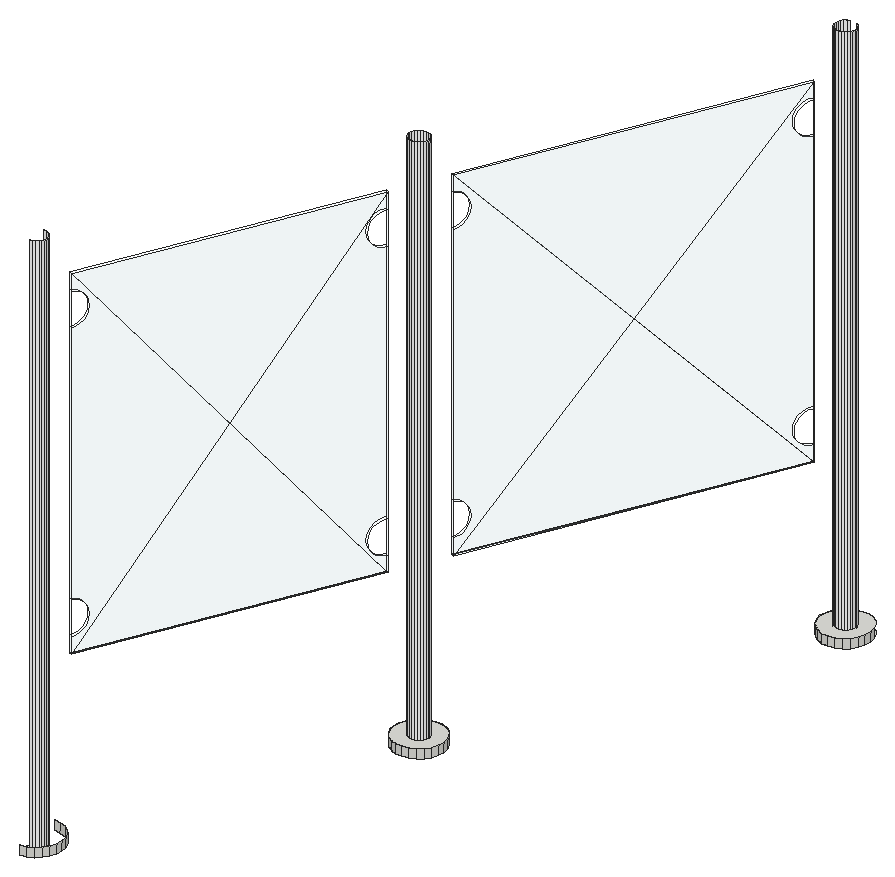
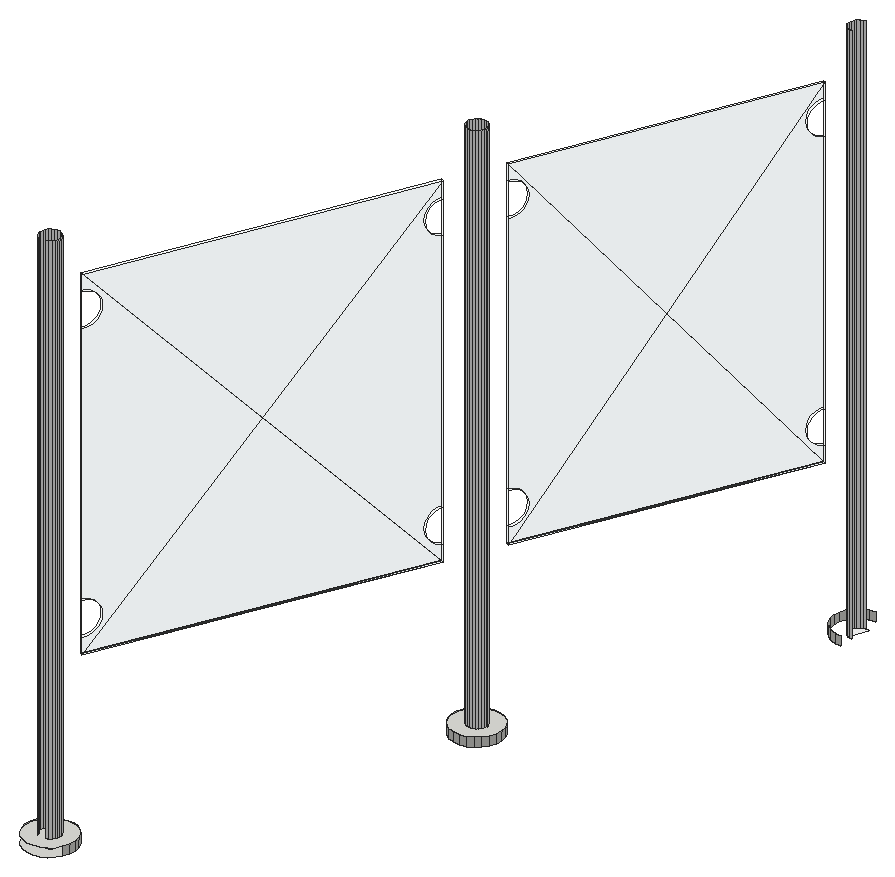
# SketchUp Ruby script. Lengths in inches.
U = 1.inch
M = Sketchup.active_model
def pt(a) = Geom::Point3d.new(a.map { |v| v * U })
def face(e, loops, mat)
  f = e.add_face(loops[0].map { |a| pt(a) })
  loops[1..].each { |l| e.add_face(l.map { |a| pt(a) }).erase! }
  f.material = f.back_material = mat if mat
  f
end
# faces: each face lists its corners as indices into pts; further lists are holes
def faces(e, pts, list, mat = nil) = list.each { |f| face(e, (f[0].is_a?(Array) ? f : [f]).map { |l| l.map { |i| pts[i] } }, mat) }
# xy, xz, yz: faces in a plane at the given z, y or x. An outline is a flat list of corners, or four numbers for a rectangle; further outlines are holes
def ring(l) = l.size == 4 ? [[l[0], l[1]], [l[2], l[1]], [l[2], l[3]], [l[0], l[3]]] : l.each_slice(2).to_a
def flat(e, list, mat, &to3) = list.each { |f| face(e, (f[0].is_a?(Array) ? f : [f]).map { |l| ring(l).map { |u, v| to3.(u, v) } }, mat) }
def xy(e, z, list, mat = nil) = flat(e, list, mat) { |x, y| [x, y, z] }
def xz(e, y, list, mat = nil) = flat(e, list, mat) { |x, z| [x, y, z] }
def yz(e, x, list, mat = nil) = flat(e, list, mat) { |y, z| [x, y, z] }
def lines(e, pts, list) = list.each { |a, b| e.add_line(pt(pts[a]), pt(pts[b])) }
# prism: a flat outline (further loops are holes) pulled along v
def prism(e, loops, v, mat = nil)
  f = face(e, loops, mat); d = Geom::Vector3d.new(v.map { |x| x * U })
  f.pushpull(f.normal.samedirection?(d) ? d.length : -d.length)
end
def box(e, o, s, mat = nil) = prism(e, [[o, [o[0] + s[0], o[1], o[2]], [o[0] + s[0], o[1] + s[1], o[2]], [o[0], o[1] + s[1], o[2]]]], [0, 0, s[2]], mat)
def at(x, y, z, deg = 0) = Geom::Transformation.translation(pt([x, y, z])) * Geom::Transformation.rotation(ORIGIN, Z_AXIS, deg.degrees)
def axes(o, x, y, z) = Geom::Transformation.new([*x, 0, *y, 0, *z, 0, *pt(o).to_a, 1])
def part(name) = M.definitions.add(name)
# library, detail: a bought-in or finely detailed component or shape, given as its bounding box
def library(name, o, s) = part(name).tap { |d| box(d.entities, o, s) }
def detail(e, o, s) = box(e.add_group.entities, o, s)
def put(e, d, t, mat = nil) = e.add_instance(d, t).tap { |i| i.material = mat if mat }
def group(e, t, mat = nil) = e.add_group.tap { |g| g.transformation = t; g.material = mat if mat }.entities
root = M.entities
M.materials.add("Glass_Safety_01").color = [204, 235, 244]
M.materials["Glass_Safety_01"].alpha = 0.1
M.materials.add("[Color_000]").color = [255, 255, 255]
xy(root,321.27,[[[898.23,660.375,898.63,660.46,899,660.64,899.31,660.92,899.53,661.26,899.66,661.65,899.6875,662.06,899.61,662.46,899.42,662.83,899.15,663.14,898.81,663.36,898.74,663.38,898.42,663.49,898,663.52,897.6,663.43,897.23,663.25,896.93,662.98,896.7,662.63,896.57,662.24,896.55,661.83,896.63,661.43,896.8125,661.0625,897.09,660.76,897.43,660.53,897.82,660.4],[898.16,661.32,898,661.33,897.87,661.37,897.84,661.38,897.7,661.47,897.6,661.59,897.52,661.74,897.49,661.9,897.5,662.07,897.55,662.22,897.64,662.36,897.76,662.47,897.91,662.54,898.07,662.58,898.24,662.57,898.37,662.52,898.39,662.51,898.53,662.42,898.64,662.3,898.71,662.15,898.75,661.99,898.74,661.83,898.68,661.67,898.59,661.53,898.47,661.43,898.32,661.35]],[897.49,660.51,897.87,661.37,897.84,661.38,897.7,661.47,897.6,661.59,897.52,661.74,897.49,661.9,897.5,662.07,897.55,662.22,897.64,662.36,897.76,662.47,897.91,662.54,898.07,662.58,898.24,662.57,898.37,662.52,898.74,663.38,898.42,663.49,898,663.52,897.6,663.43,897.23,663.25,896.93,662.98,896.7,662.63,896.57,662.24,896.55,661.83,896.63,661.43,896.8125,661.0625,897.09,660.76,897.43,660.53],[897.87,661.37,898.37,662.52,898.24,662.57,898.07,662.58,897.91,662.54,897.76,662.47,897.64,662.36,897.55,662.22,897.5,662.07,897.49,661.9,897.52,661.74,897.6,661.59,897.7,661.47,897.84,661.38],[[908.17,683.21,908.58,683.29,908.95,683.48,909.25,683.75,909.48,684.09,909.61,684.48,909.63,684.89,909.55,685.3,909.37,685.66,909.09,685.97,908.75,686.2,908.6875,686.22,908.36,686.33,907.95,686.35,907.55,686.27,907.18,686.09,906.87,685.8125,906.65,685.47,906.52,685.08,906.49,684.67,906.57,684.27,906.76,683.9,907.03,683.59,907.375,683.36,907.4375,683.34,907.76,683.23],[908.11,684.15,907.94,684.16,907.8125,684.21,907.79,684.21,907.65,684.3,907.54,684.43,907.47,684.57,907.43,684.74,907.44,684.9,907.5,685.06,907.59,685.19,907.71,685.3,907.86,685.375,908.02,685.41,908.18,685.4,908.3125,685.36,908.34,685.35,908.47,685.26,908.58,685.13,908.66,684.99,908.69,684.83,908.68,684.66,908.63,684.51,908.54,684.37,908.42,684.26,908.27,684.1875]],[907.4375,683.34,907.8125,684.21,907.79,684.21,907.65,684.3,907.54,684.43,907.47,684.57,907.43,684.74,907.44,684.9,907.5,685.06,907.59,685.19,907.71,685.3,907.86,685.375,908.02,685.41,908.18,685.4,908.3125,685.36,908.6875,686.22,908.36,686.33,907.95,686.35,907.55,686.27,907.18,686.09,906.87,685.8125,906.65,685.47,906.52,685.08,906.49,684.67,906.57,684.27,906.76,683.9,907.03,683.59,907.375,683.36],
  [907.79,684.21,907.8125,684.21,908.3125,685.36,908.18,685.4,908.02,685.41,907.86,685.375,907.71,685.3,907.59,685.19,907.5,685.06,907.44,684.9,907.43,684.74,907.47,684.57,907.54,684.43,907.65,684.3]])
xy(root,321.27,[[889.26,640.88,889.42,640.91,889.57,640.99,889.69,641.1,889.78,641.23,889.83,641.39,889.84,641.55,889.8125,641.71,889.74,641.86,889.63,641.98,889.49,642.07,889.47,642.08,888.97,640.93,889.1,640.89],[898.16,661.32,898.32,661.35,898.47,661.43,898.59,661.53,898.68,661.67,898.74,661.83,898.75,661.99,898.71,662.15,898.64,662.3,898.53,662.42,898.39,662.51,898.37,662.52,897.87,661.37,898,661.33],[908.11,684.15,908.27,684.1875,908.42,684.26,908.54,684.37,908.63,684.51,908.68,684.66,908.69,684.83,908.66,684.99,908.58,685.13,908.47,685.26,908.34,685.35,908.3125,685.36,907.8125,684.21,907.94,684.16]],"[Color_000]")
xy(root,321.86,[[898.23,660.375,898.63,660.46,899,660.64,899.31,660.92,899.53,661.26,899.66,661.65,899.6875,662.06,899.61,662.46,899.42,662.83,899.15,663.14,898.81,663.36,898.42,663.49,898,663.52,897.6,663.43,897.23,663.25,896.93,662.98,896.7,662.63,896.57,662.24,896.55,661.83,896.63,661.43,896.8125,661.0625,897.09,660.76,897.43,660.53,897.82,660.4],[908.17,683.21,908.58,683.29,908.95,683.48,909.25,683.75,909.48,684.09,909.61,684.48,909.63,684.89,909.55,685.3,909.37,685.66,909.09,685.97,908.75,686.2,908.36,686.33,907.95,686.35,907.55,686.27,907.18,686.09,906.87,685.8125,906.65,685.47,906.52,685.08,906.49,684.67,906.57,684.27,906.76,683.9,907.03,683.59,907.375,683.36,907.76,683.23]])
xy(root,331.9,[[890.09,643.27,889.91,643.35,897.49,660.26],[889.91,643.35,897.31,660.34,897.49,660.26],[898.99,663.71,898.8125,663.79,907.43,683.08],[898.8125,663.79,907.25,683.16,907.43,683.08]],"Glass_Safety_01")
p = [[889.33,639.9375,321.27],[889.73,640.02,321.27],[889.73,640.02,321.86],[889.33,639.9375,321.86],[890.1,640.2,321.27],[890.1,640.2,321.86],
  [890.41,640.48,321.27],[890.41,640.48,321.86],[890.63,640.82,321.27],[890.63,640.82,321.86],[890.76,641.21,321.27],[890.76,641.21,321.86],
  [889.26,640.88,321.27],[889.42,640.91,321.27],[889.42,640.91,357.27],[889.26,640.88,357.27],[889.57,640.99,321.27],[889.57,640.99,357.27],
  [889.69,641.1,321.27],[889.69,641.1,357.27],[889.78,641.23,321.27],[889.78,641.23,357.27],[889.83,641.39,321.27],[889.83,641.39,357.27],
  [890.79,641.62,321.27],[890.79,641.62,321.86],[889.84,641.55,321.27],[889.84,641.55,357.27],[889.8125,641.71,321.27],[889.8125,641.71,357.27],
  [890.7,642.02,321.27],[890.7,642.02,321.86],[889.74,641.86,321.27],[889.74,641.86,357.27],[889.63,641.98,321.27],[889.63,641.98,357.27],
  [889.49,642.07,321.27],[889.49,642.07,357.27],[890.52,642.39,321.27],[890.52,642.39,321.86],[889.33,642.125,321.27],[889.17,642.14,321.27],
  [889.17,642.14,357.27],[889.33,642.125,357.27],[889.47,642.08,321.27],[890.25,642.7,321.27],[890.25,642.7,321.86],[889.9,642.92,321.27],
  [889.9,642.92,321.86],[889.84,642.94,321.27],[889.51,643.05,321.27],[889.51,643.05,321.86],[889.1,643.08,321.27],[889.1,643.08,321.86],
  [897.43,660.53,321.27],[897.49,660.51,321.27],[897.82,660.4,321.27],[897.82,660.4,321.86],[897.43,660.53,321.86],[898.23,660.375,321.27],
  [898.23,660.375,321.86],[898.63,660.46,321.27],[898.63,660.46,321.86],[897.09,660.76,321.27],[897.09,660.76,321.86],[899,660.64,321.27],
  [899,660.64,321.86],[899.31,660.92,321.27],[899.31,660.92,321.86],[896.8125,661.0625,321.27],[896.8125,661.0625,321.86],[899.53,661.26,321.27],
  [899.53,661.26,321.86],[896.63,661.43,321.27],[896.63,661.43,321.86],[897.84,661.38,321.27],[897.87,661.37,321.27],[898,661.33,321.27],
  [898,661.33,357.27],[897.84,661.38,357.27],[898.16,661.32,321.27],[898.16,661.32,357.27],[898.32,661.35,321.27],[898.32,661.35,357.27],
  [899.66,661.65,321.27],[899.66,661.65,321.86],[896.55,661.83,321.27],[896.55,661.83,321.86],[897.7,661.47,321.27],[897.7,661.47,357.27],
  [898.47,661.43,321.27],[898.47,661.43,357.27],[898.59,661.53,321.27],[898.59,661.53,357.27],[897.6,661.59,321.27],[897.6,661.59,357.27],
  [898.68,661.67,321.27],[898.68,661.67,357.27],[897.52,661.74,321.27],[897.52,661.74,357.27],[899.6875,662.06,321.27],[899.6875,662.06,321.86],
  [897.49,661.9,321.27],[897.49,661.9,357.27],[898.74,661.83,321.27],[898.74,661.83,357.27],[896.57,662.24,321.27],[896.57,662.24,321.86],
  [898.75,661.99,321.27],[898.75,661.99,357.27],[897.5,662.07,321.27],[897.5,662.07,357.27],[898.71,662.15,321.27],[898.71,662.15,357.27],
  [897.55,662.22,321.27],[897.55,662.22,357.27],[899.61,662.46,321.27],[899.61,662.46,321.86],[896.7,662.63,321.27],[896.7,662.63,321.86],
  [897.64,662.36,321.27],[897.64,662.36,357.27],[898.64,662.3,321.27],[898.64,662.3,357.27],[898.53,662.42,321.27],[898.53,662.42,357.27],
  [897.76,662.47,321.27],[897.76,662.47,357.27],[898.39,662.51,321.27],[898.39,662.51,357.27],[897.91,662.54,321.27],[897.91,662.54,357.27],
  [898.07,662.58,321.27],[898.07,662.58,357.27],[898.37,662.52,321.27],[898.24,662.57,321.27],[898.24,662.57,357.27],[899.42,662.83,321.27],
  [899.42,662.83,321.86],[896.93,662.98,321.27],[896.93,662.98,321.86],[899.15,663.14,321.27],[899.15,663.14,321.86],[897.23,663.25,321.27],
  [897.23,663.25,321.86],[898.81,663.36,321.27],[898.81,663.36,321.86],[897.6,663.43,321.27],[897.6,663.43,321.86],[898,663.52,321.27],
  [898,663.52,321.86],[898.74,663.38,321.27],[898.42,663.49,321.27],[898.42,663.49,321.86],[907.375,683.36,321.27],[907.4375,683.34,321.27],
  [907.76,683.23,321.27],[907.76,683.23,321.86],[907.375,683.36,321.86],[908.17,683.21,321.27],[908.17,683.21,321.86],[908.58,683.29,321.27],
  [908.58,683.29,321.86],[908.95,683.48,321.27],[908.95,683.48,321.86],[907.03,683.59,321.27],[907.03,683.59,321.86],[909.25,683.75,321.27],
  [909.25,683.75,321.86],[906.76,683.9,321.27],[906.76,683.9,321.86],[909.48,684.09,321.27],[909.48,684.09,321.86],[906.57,684.27,321.27],
  [906.57,684.27,321.86],[909.61,684.48,321.27],[909.61,684.48,321.86],[907.65,684.3,321.27],[907.79,684.21,321.27],[907.79,684.21,357.27],
  [907.65,684.3,357.27],[907.8125,684.21,321.27],[907.94,684.16,321.27],[907.94,684.16,357.27],[908.11,684.15,321.27],[908.11,684.15,357.27],
  [908.27,684.1875,321.27],[908.27,684.1875,357.27],[908.42,684.26,321.27],[908.42,684.26,357.27],[906.49,684.67,321.27],[906.49,684.67,321.86],
  [907.54,684.43,321.27],[907.54,684.43,357.27],[908.54,684.37,321.27],[908.54,684.37,357.27],[907.47,684.57,321.27],[907.47,684.57,357.27],
  [908.63,684.51,321.27],[908.63,684.51,357.27],[908.68,684.66,321.27],[908.68,684.66,357.27],[909.63,684.89,321.27],[909.63,684.89,321.86],
  [907.43,684.74,321.27],[907.43,684.74,357.27],[906.52,685.08,321.27],[906.52,685.08,321.86],[907.44,684.9,321.27],[907.44,684.9,357.27],
  [908.69,684.83,321.27],[908.69,684.83,357.27],[908.66,684.99,321.27],[908.66,684.99,357.27],[907.5,685.06,321.27],[907.5,685.06,357.27],
  [909.55,685.3,321.27],[909.55,685.3,321.86],[908.58,685.13,321.27],[908.58,685.13,357.27],[906.65,685.47,321.27],[906.65,685.47,321.86],
  [907.59,685.19,321.27],[907.59,685.19,357.27],[908.47,685.26,321.27],[908.47,685.26,357.27],[907.71,685.3,321.27],[907.71,685.3,357.27],
  [907.86,685.375,321.27],[907.86,685.375,357.27],[908.34,685.35,321.27],[908.34,685.35,357.27],[889.91,643.35,331.9],[890.09,643.27,331.9],
  [890.09,643.27,333],[890.09,643.27,335.125],[890.09,643.27,351.28],[890.09,643.27,353.41],[890.09,643.27,354.51],[889.91,643.35,354.51],
  [889.91,643.35,353.41],[889.91,643.35,351.28],[889.91,643.35,335.125],[889.91,643.35,333],[890.2,643.53,335.09],[890.3,643.76,334.98],
  [890.39,643.96,334.8125],[890.46,644.12,334.59],[890.5,644.21,334.34],[890.52,644.25,334.0625],[890.5,644.21,333.79],[890.46,644.12,333.53],
  [890.39,643.96,333.3125],[890.3,643.76,333.14],[890.2,643.53,333.04],[897.49,660.26,354.51],[890.2,643.53,353.37],[890.3,643.76,353.27],
  [890.39,643.96,353.1],[890.46,644.12,352.88],[890.5,644.21,352.62],[890.52,644.25,352.35],[890.5,644.21,352.07],[890.46,644.12,351.8125],
  [890.39,643.96,351.59],[890.3,643.76,351.43],[890.2,643.53,351.32],[897.49,660.26,331.9],[897.49,660.26,333],[897.42,660.1,333],
  [897.3125,659.85,333.04],[897.21,659.62,333.14],[897.12,659.41,333.3125],[897.05,659.26,333.53],[897.01,659.16,333.79],[897,659.13,334.0625],
  [897.01,659.16,334.34],[897.05,659.26,334.59],[897.12,659.41,334.8125],[897.21,659.62,334.98],[897.3125,659.85,335.09],[897.42,660.1,335.125],
  [897.49,660.26,335.125],[897.49,660.26,351.28],[897.42,660.1,351.28],[897.3125,659.85,351.32],[897.21,659.62,351.43],[897.12,659.41,351.59],
  [897.05,659.26,351.8125],[897.01,659.16,352.07],[897,659.13,352.35],[897.01,659.16,352.62],[897.05,659.26,352.88],[897.12,659.41,353.1],
  [897.21,659.62,353.27],[897.3125,659.85,353.37],[897.42,660.1,353.41],[897.49,660.26,353.41],[890.02,643.6,333.04],[890.125,643.84,333.14],
  [890.21,644.04,333.3125],[890.28,644.2,333.53],[890.32,644.29,333.79],[890.34,644.33,334.0625],[890.32,644.29,334.34],[890.28,644.2,334.59],
  [890.21,644.04,334.8125],[890.125,643.84,334.98],[890.02,643.6,335.09],[890.02,643.6,351.32],[890.125,643.84,351.43],[890.21,644.04,351.59],
  [890.28,644.2,351.8125],[890.32,644.29,352.07],[890.34,644.33,352.35],[890.32,644.29,352.62],[890.28,644.2,352.88],[890.21,644.04,353.1],
  [890.125,643.84,353.27],[890.02,643.6,353.37],[897.31,660.34,331.9],[897.31,660.34,351.28],[897.31,660.34,335.125],[897.24,660.18,335.125],
  [897.13,659.93,335.09],[897.03,659.69,334.98],[896.94,659.49,334.8125],[896.875,659.34,334.59],[896.83,659.24,334.34],[896.82,659.21,334.0625],
  [896.83,659.24,333.79],[896.875,659.34,333.53],[896.94,659.49,333.3125],[897.03,659.69,333.14],[897.13,659.93,333.04],[897.24,660.18,333],
  [897.31,660.34,333],[897.31,660.34,354.51],[897.31,660.34,353.41],[897.24,660.18,353.41],[897.13,659.93,353.37],[897.03,659.69,353.27],
  [896.94,659.49,353.1],[896.875,659.34,352.88],[896.83,659.24,352.62],[896.82,659.21,352.35],[896.83,659.24,352.07],[896.875,659.34,351.8125],
  [896.94,659.49,351.59],[897.03,659.69,351.43],[897.13,659.93,351.32],[897.24,660.18,351.28],[898.8125,663.79,331.9],[898.99,663.71,331.9],
  [898.99,663.71,333],[898.99,663.71,335.125],[898.99,663.71,351.28],[898.99,663.71,353.41],[898.99,663.71,354.51],[898.8125,663.79,354.51],
  [898.8125,663.79,353.41],[898.8125,663.79,351.28],[898.8125,663.79,335.125],[898.8125,663.79,333],[899.1,663.96,335.09],[899.21,664.2,334.98],
  [899.29,664.4,334.8125],[899.36,664.56,334.59],[899.4,664.65,334.34],[899.42,664.6875,334.0625],[899.4,664.65,333.79],[899.36,664.56,333.53],
  [899.29,664.4,333.3125],[899.21,664.2,333.14],[899.1,663.96,333.04],[907.43,683.08,354.51],[899.1,663.96,353.37],[899.21,664.2,353.27],
  [899.29,664.4,353.1],[899.36,664.56,352.88],[899.4,664.65,352.62],[899.42,664.6875,352.35],[899.4,664.65,352.07],[899.36,664.56,351.8125],
  [899.29,664.4,351.59],[899.21,664.2,351.43],[899.1,663.96,351.32],[907.43,683.08,331.9],[907.43,683.08,333],[907.37,682.9375,333],
  [907.26,682.68,333.04],[907.15,682.45,333.14],[907.07,682.25,333.3125],[907,682.09,333.53],[906.96,682,333.79],[906.94,681.96,334.0625],
  [906.96,682,334.34],[907,682.09,334.59],[907.07,682.25,334.8125],[907.15,682.45,334.98],[907.26,682.68,335.09],[907.37,682.9375,335.125],
  [907.43,683.08,335.125],[907.43,683.08,351.28],[907.37,682.9375,351.28],[907.26,682.68,351.32],[907.15,682.45,351.43],[907.07,682.25,351.59],
  [907,682.09,351.8125],[906.96,682,352.07],[906.94,681.96,352.35],[906.96,682,352.62],[907,682.09,352.88],[907.07,682.25,353.1],
  [907.15,682.45,353.27],[907.26,682.68,353.37],[907.37,682.9375,353.41],[907.43,683.08,353.41],[898.92,664.04,333.04],[899.03,664.28,333.14],
  [899.11,664.48,333.3125],[899.18,664.63,333.53],[899.22,664.73,333.79],[899.24,664.77,334.0625],[899.22,664.73,334.34],[899.18,664.63,334.59],
  [899.11,664.48,334.8125],[899.03,664.28,334.98],[898.92,664.04,335.09],[898.92,664.04,351.32],[899.03,664.28,351.43],[899.11,664.48,351.59],
  [899.18,664.63,351.8125],[899.22,664.73,352.07],[899.24,664.77,352.35],[899.22,664.73,352.62],[899.18,664.63,352.88],[899.11,664.48,353.1],
  [899.03,664.28,353.27],[898.92,664.04,353.37],[907.25,683.16,331.9],[907.25,683.16,351.28],[907.25,683.16,335.125],[907.1875,683.02,335.125],
  [907.08,682.76,335.09],[906.97,682.53,334.98],[906.89,682.33,334.8125],[906.82,682.17,334.59],[906.78,682.07,334.34],[906.76,682.04,334.0625],
  [906.78,682.07,333.79],[906.82,682.17,333.53],[906.89,682.33,333.3125],[906.97,682.53,333.14],[907.08,682.76,333.04],[907.1875,683.02,333],
  [907.25,683.16,333],[907.25,683.16,354.51],[907.25,683.16,353.41],[907.1875,683.02,353.41],[907.08,682.76,353.37],[906.97,682.53,353.27],
  [906.89,682.33,353.1],[906.82,682.17,352.88],[906.78,682.07,352.62],[906.76,682.04,352.35],[906.78,682.07,352.07],[906.82,682.17,351.8125],
  [906.89,682.33,351.59],[906.97,682.53,351.43],[907.08,682.76,351.32],[907.1875,683.02,351.28]]
faces(root,p,[[0,1,2,3],[1,4,5,2],[4,6,7,5],[6,8,9,7],[8,10,11,9],[10,24,25,11],[24,30,31,25],[30,38,39,31],
  [38,45,46,39],[45,47,48,46],[47,49,50,51,48],[50,52,53,51],[54,55,56,57,58],[56,59,60,57],[59,61,62,60],[63,54,58,64],
  [61,65,66,62],[65,67,68,66],[69,63,64,70],[67,71,72,68],[73,69,70,74],[71,84,85,72],[86,73,74,87],[84,100,101,85],
  [106,86,87,107],[100,116,117,101],[118,106,107,119],[116,137,138,117],[139,118,119,140],[137,141,142,138],[143,139,140,144],[141,145,146,142],
  [147,143,144,148],[149,147,148,150],[145,151,152,153,146],[152,149,150,153],[154,155,156,157,158],[156,159,160,157],[159,161,162,160],[161,163,164,162],
  [165,154,158,166],[163,167,168,164],[169,165,166,170],[167,171,172,168],[173,169,170,174],[171,175,176,172],[190,173,174,191],[175,202,203,176],
  [206,190,191,207],[202,216,217,203],[220,206,207,221]])
faces(root,p,[[12,13,14,15],[13,16,17,14],[16,18,19,17],[18,20,21,19],[20,22,23,21],[22,26,27,23],[26,28,29,27],[28,32,33,29],
  [32,34,35,33],[34,36,37,35],[40,41,42,43],[36,44,40,43,37],[75,76,77,78,79],[77,80,81,78],[80,82,83,81],[88,75,79,89],
  [82,90,91,83],[90,92,93,91],[94,88,89,95],[92,96,97,93],[98,94,95,99],[102,98,99,103],[96,104,105,97],[104,108,109,105],
  [110,102,103,111],[108,112,113,109],[114,110,111,115],[120,114,115,121],[112,122,123,113],[122,124,125,123],[126,120,121,127],[124,128,129,125],
  [130,126,127,131],[132,130,131,133],[128,134,135,136,129],[135,132,133,136],[177,178,179,180],[178,181,182,183,179],[182,184,185,183],[184,186,187,185],
  [186,188,189,187],[192,177,180,193],[188,194,195,189],[196,192,193,197],[194,198,199,195],[198,200,201,199],[204,196,197,205],[208,204,205,209],
  [200,210,211,201],[210,212,213,211],[214,208,209,215],[212,218,219,213],[222,214,215,223],[218,224,225,219],[226,222,223,227],[228,226,227,229],
  [224,230,231,225]],"[Color_000]")
faces(root,p,[[232,233,234,235,236,237,238,239,240,241,242,243],[236,235,244,245,246,247,248,249,250,251,252,253,254,234,233,255,238,237,256,257,258,259,260,261,262,263,264,265,266],[267,268,269,270,271,272,273,274,275,276,277,278,279,280,281,282,283,284,285,286,287,288,289,290,291,292,293,294,295,296,297,255,233],[232,243,298,299,300,301,302,303,304,305,306,307,308,242,241,309,310,311,312,313,314,315,316,317,318,319,240,239,320],[321,322,323,324,325,326,327,328,329,330,331,332,333,334,335,336,320,239,337,338,339,340,341,342,343,344,345,346,347,348,349,350,351],[267,320,336,322,321,338,337,255,297,283,282,268],[352,353,354,355,356,357,358,359,360,361,362,363],[356,355,364,365,366,367,368,369,370,371,372,373,374,354,353,375,358,357,376,377,378,379,380,381,382,383,384,385,386],
  [387,388,389,390,391,392,393,394,395,396,397,398,399,400,401,402,403,404,405,406,407,408,409,410,411,412,413,414,415,416,417,375,353],[352,363,418,419,420,421,422,423,424,425,426,427,428,362,361,429,430,431,432,433,434,435,436,437,438,439,360,359,440],[441,442,443,444,445,446,447,448,449,450,451,452,453,454,455,456,440,359,457,458,459,460,461,462,463,464,465,466,467,468,469,470,471],[387,440,456,442,441,458,457,375,417,403,402,388]],"Glass_Safety_01")
